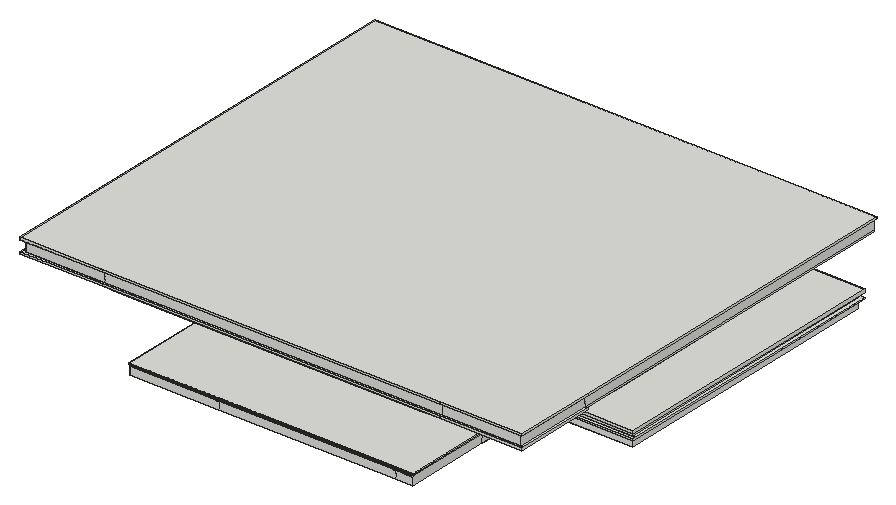
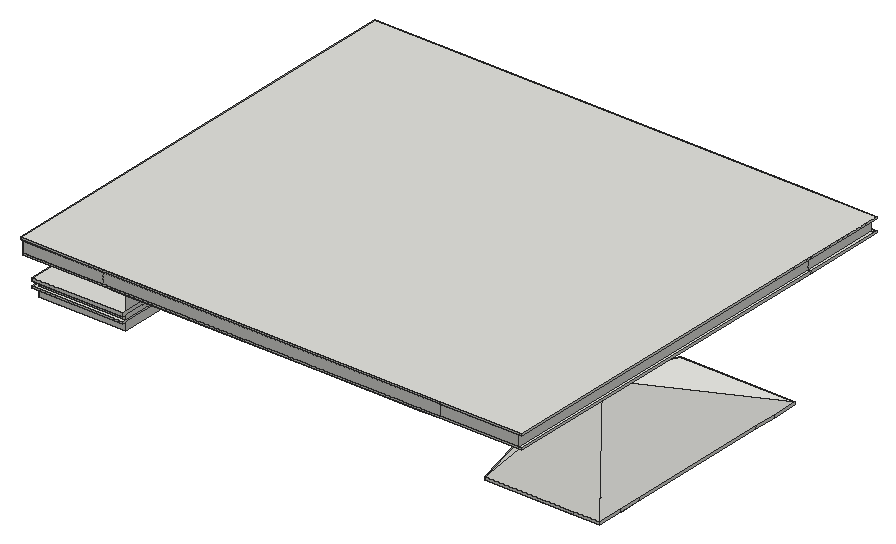
# SketchUp Ruby script. Lengths in inches.
U = 1.inch
M = Sketchup.active_model
def pt(a) = Geom::Point3d.new(a.map { |v| v * U })
def face(e, loops, mat)
  f = e.add_face(loops[0].map { |a| pt(a) })
  loops[1..].each { |l| e.add_face(l.map { |a| pt(a) }).erase! }
  f.material = f.back_material = mat if mat
  f
end
# faces: each face lists its corners as indices into pts; further lists are holes
def faces(e, pts, list, mat = nil) = list.each { |f| face(e, (f[0].is_a?(Array) ? f : [f]).map { |l| l.map { |i| pts[i] } }, mat) }
# xy, xz, yz: faces in a plane at the given z, y or x. An outline is a flat list of corners, or four numbers for a rectangle; further outlines are holes
def ring(l) = l.size == 4 ? [[l[0], l[1]], [l[2], l[1]], [l[2], l[3]], [l[0], l[3]]] : l.each_slice(2).to_a
def flat(e, list, mat, &to3) = list.each { |f| face(e, (f[0].is_a?(Array) ? f : [f]).map { |l| ring(l).map { |u, v| to3.(u, v) } }, mat) }
def xy(e, z, list, mat = nil) = flat(e, list, mat) { |x, y| [x, y, z] }
def xz(e, y, list, mat = nil) = flat(e, list, mat) { |x, z| [x, y, z] }
def yz(e, x, list, mat = nil) = flat(e, list, mat) { |y, z| [x, y, z] }
def lines(e, pts, list) = list.each { |a, b| e.add_line(pt(pts[a]), pt(pts[b])) }
# prism: a flat outline (further loops are holes) pulled along v
def prism(e, loops, v, mat = nil)
  f = face(e, loops, mat); d = Geom::Vector3d.new(v.map { |x| x * U })
  f.pushpull(f.normal.samedirection?(d) ? d.length : -d.length)
end
def box(e, o, s, mat = nil) = prism(e, [[o, [o[0] + s[0], o[1], o[2]], [o[0] + s[0], o[1] + s[1], o[2]], [o[0], o[1] + s[1], o[2]]]], [0, 0, s[2]], mat)
def at(x, y, z, deg = 0) = Geom::Transformation.translation(pt([x, y, z])) * Geom::Transformation.rotation(ORIGIN, Z_AXIS, deg.degrees)
def axes(o, x, y, z) = Geom::Transformation.new([*x, 0, *y, 0, *z, 0, *pt(o).to_a, 1])
def part(name) = M.definitions.add(name)
# library, detail: a bought-in or finely detailed component or shape, given as its bounding box
def library(name, o, s) = part(name).tap { |d| box(d.entities, o, s) }
def detail(e, o, s) = box(e.add_group.entities, o, s)
def put(e, d, t, mat = nil) = e.add_instance(d, t).tap { |i| i.material = mat if mat }
def group(e, t, mat = nil) = e.add_group.tap { |g| g.transformation = t; g.material = mat if mat }.entities
root = M.entities
M.materials.add("Glass Thin Clear 001").color = [255, 250, 250]
M.materials["Glass Thin Clear 001"].alpha = 0.1
M.materials.add("[Color M07]").color = [58, 58, 58]
xy(root,335.4,[[79.0625,304.1875,79.0625,318.3125,79.875,318.3125,79.875,305,93.1875,305,93.1875,304.1875],[93.1875,304.1875,94,305],[94,304.1875,142,305],[79.875,305,93.1875,318.3125],[93.1875,305,94,318.3125],
  [94,305,142,318.3125],[79.0625,318.3125,79.875,331.125],[79.875,318.3125,93.1875,319.125],[93.1875,318.3125,94,319.125],[94,318.3125,142,319.125],
  [79.875,319.125,93.1875,331.125],[93.1875,319.125,94,331.125],[94,319.125,142,423.25],[79.0625,331.125,79.875,411.25],[79.875,331.125,93.1875,411.25],
  [93.1875,331.125,94,411.25],[79.0625,411.25,79.875,423.25],[79.875,411.25,93.1875,423.25],[93.1875,411.25,94,423.25],[79.0625,423.25,79.875,424.0625],
  [79.875,423.25,93.1875,424.0625],[93.1875,423.25,94,424.0625],[94,423.25,142,424.0625],[79.0625,424.0625,79.0625,438.1875,93.1875,438.1875,93.1875,437.375,79.875,437.375,79.875,424.0625],[79.875,424.0625,93.1875,437.375],
  [93.1875,424.0625,94,437.375],[94,424.0625,142,437.375],[93.1875,437.375,142,438.1875]])
xy(root,350.5625,[[326.84,298.82,374.84,453.63]])
xy(root,351.07,[[169.81,269.93,207.43,270.37],[169.81,270.37,207.43,272.05]],"[Color M07]")
xy(root,351.46,[[241.62,260.1875,243.38,264.4375],[261.3,260.1875,263.07,264.4375],[283.05,260.1875,284.82,264.4375],[308.3125,260.1875,310.08,264.4375]])
xy(root,351.46,[[223.93,260.1875,241.62,261.1875],[243.38,260.1875,261.3,261.1875],[263.07,260.1875,283.05,261.1875],[284.82,260.1875,308.3125,261.1875],[310.08,260.1875,317.84,261.1875],
  [317.84,260.1875,323.73,261.1875],[223.93,261.1875,241.62,264.4375],[243.38,261.1875,261.3,264.4375],[263.07,261.1875,283.05,264.4375],[284.82,261.1875,308.3125,264.4375],
  [310.08,261.1875,317.84,264.4375],[317.84,261.1875,323.73,264.4375]],"[Color M07]")
xy(root,354.57,[[171.8125,207.6875,220.8125,255.6875],[220.8125,207.6875,317.84,255.6875],[317.84,207.6875,326.84,255.6875],[171.8125,255.6875,209.4375,264.6875],[220.8125,255.6875,317.84,260.1875],
  [317.84,255.6875,326.84,260.1875],[220.8125,264.4375,317.84,264.6875],[317.84,264.4375,326.84,264.6875],[171.8125,264.6875,171.8125,271.43,173.3125,271.43,173.3125,269.93,209.4375,269.93,209.4375,264.6875],[171.8125,271.43,171.8125,280.43,209.4375,280.43,209.4375,272.05,173.3125,272.05,173.3125,271.43]])
xy(root,354.57,[[220.8125,260.1875,317.84,262.625],[317.84,260.1875,326.84,262.625],[220.8125,262.625,317.84,264.4375],[317.84,262.625,326.84,264.4375],[173.3125,269.93,209.4375,271.43],
  [209.4375,269.93,210.9375,271.43],[173.3125,271.43,209.4375,272.05],[209.4375,271.43,210.9375,272.05]],"[Color M07]")
xy(root,354.9375,[[326.84,296.95,376.71,298.82],[326.84,298.82,374.84,453.63],[374.84,298.82,376.71,455.51],[326.84,453.63,374.84,455.51]])
xy(root,355.8125,[[326.84,296.95,376.71,298.82],[326.84,298.82,374.84,453.63],[374.84,298.82,376.71,455.51],[326.84,453.63,374.84,455.51]])
xy(root,356.5,[[169.62,269.93,169.81,270.37],[169.62,270.37,169.81,272.05]],"[Color M07]")
xy(root,356.87,[[166.4375,269.93,168.4375,272.05]])
xy(root,356.87,[[145.94,269.93,166.4375,270.37],[168.4375,269.93,169.62,270.37],[145.94,270.37,166.4375,272.05],[168.4375,270.37,169.62,272.05]],"[Color M07]")
xy(root,357.54,[[142,273.2,142.4375,280.43],[142.4375,273.2,144.125,280.43],[142,280.43,142.4375,289.29],[142.4375,280.43,144.125,289.29]],"[Color M07]")
xy(root,358.3125,[[326.84,296.95,376.71,298.82],[326.84,298.82,374.84,453.63],[374.84,298.82,376.71,455.51],[326.84,453.63,374.84,455.51]])
xy(root,359,[[171.625,207.5625,171.8125,280.43],[171.8125,207.5625,220.8125,207.6875],[220.8125,207.5625,317.84,207.6875],[317.84,207.5625,326.84,207.6875]])
xy(root,359.1875,[[171.8125,207.6875,326.84,255.6875]])
xy(root,359.4375,[[171.625,207.5625,209.5625,207.5625,209.5625,207.8125,171.9375,207.8125,171.9375,255.6875,171.8125,255.6875,171.8125,280.43,171.625,280.43],[209.5625,207.5625,220.8125,207.8125],[220.8125,207.5625,317.84,207.8125],[317.84,207.5625,326.84,207.8125],[171.9375,207.8125,326.71,255.6875],
  [326.71,207.8125,326.84,255.6875]])
xy(root,360,[[171.625,207.5,171.625,271.43,171.8125,271.43,171.8125,255.6875,171.9375,255.6875,171.9375,207.8125,209.5625,207.8125,209.5625,207.5],[209.5625,207.5,220.8125,207.8125],[220.8125,207.5,317.84,207.8125],[317.84,207.5,327.03,207.8125],[171.9375,207.8125,326.71,255.6875],
  [326.71,207.8125,327.03,255.6875],[171.8125,255.6875,171.9375,264.6875],[171.9375,255.6875,326.84,264.6875],[171.8125,264.6875,171.9375,271.43],[171.9375,264.6875,171.9375,271.43,173.125,271.43,173.125,269.93,173.3125,269.93,173.3125,271.43,220.8125,271.43,220.8125,264.6875],
  [220.8125,264.6875,317.84,271.43],[317.84,264.6875,326.84,271.43],[171.625,271.43,171.8125,280.43],[326.84,296.95,376.71,455.51]])
xy(root,360,[[173.125,269.93,173.3125,271.43],[173.125,271.43,173.3125,272.05]],"[Color M07]")
xy(root,360.375,[[171.625,271.43,173.125,272.05],[173.25,271.43,209.4375,272.18],[209.4375,271.43,211.0625,272.18],[211.0625,271.43,211.0625,272.18,209.4375,272.18,209.4375,280.43,220.8125,280.43,220.8125,271.43],[220.8125,271.43,326.84,280.43],
  [171.625,272.18,209.4375,280.43]])
xy(root,360.375,[[142,269.8,143.625,269.93],[143.625,269.8,144.375,269.93],[144.375,269.8,144.375,269.93,173.125,269.93,173.125,271.43,173.25,271.43,173.25,269.8],[173.25,269.8,211.0625,271.43],[142,269.93,143.5,271.43],
  [143.5,269.93,143.625,271.43],[143.625,269.93,144.125,271.43],[144.125,269.93,144.375,271.43],[144.375,269.93,173.125,271.43],[142,271.43,143.5,280.43],
  [143.5,271.43,143.625,280.43],[143.625,271.43,144.125,280.43],[144.125,271.43,144.375,272.05],[144.375,271.43,144.375,272.05,171.625,272.05,171.625,272.18,173.25,272.18,173.25,271.43,173.125,271.43,173.125,272.05,171.625,272.05,171.625,271.43],[144.125,272.05,144.375,280.43],
  [144.375,272.05,171.625,272.18],[142,280.43,143.5,292.12],[143.5,280.43,143.625,292.12],[143.625,280.43,144.125,292.12],[144.125,280.43,144.375,292.12]],"[Color M07]")
xy(root,360.6875,[[171.625,207.5,327.03,207.5,327.03,255.6875,326.84,255.6875,326.84,271.43,171.625,271.43]])
xy(root,361.53,[[142,271.52,142.5625,280.43],[142.5625,271.52,144.375,280.43],[142,280.43,142.5625,290.97],[142.5625,280.43,144.375,290.97]],"[Color M07]")
xy(root,361.68,[[143.86,269.8,144.375,270.37],[166.5625,269.8,168.5625,272.18]])
xy(root,361.68,[[144.375,269.8,166.5625,270.37],[168.5625,269.8,173.25,270.37],[173.25,269.8,209.76,270.37],[144.375,270.37,166.5625,272.18],[168.5625,270.37,173.25,272.18],
  [173.25,270.37,209.76,272.18]],"[Color M07]")
xy(root,366.64,[[143.86,269.8,144.375,270.37],[166.5625,269.8,168.5625,272.18]])
xy(root,366.64,[[144.375,269.8,166.5625,270.37],[168.5625,269.8,209.76,270.37],[144.375,270.37,166.5625,272.18],[168.5625,270.37,209.76,272.18]],"[Color M07]")
xy(root,366.79,[[142,271.52,142.5625,280.43],[142.5625,271.52,144.375,280.43],[142,280.43,142.5625,290.97],[142.5625,280.43,144.375,290.97]],"[Color M07]")
xy(root,367.9375,[[144.375,272.18,144.375,292.12,151,292.12,151,280.43,209.4375,280.43,209.4375,272.18]])
xy(root,367.9375,[[142,269.8,143.625,271.43],[143.625,269.8,144.375,271.43],[144.375,269.8,211.0625,271.43],[142,271.43,143.625,280.43],[143.625,271.43,144.375,280.43],
  [209.4375,271.43,211.0625,272.18],[142,280.43,143.625,292.12],[143.625,280.43,144.375,292.12]],"[Color M07]")
xy(root,379.5625,[[96.8125,226.24,142,271.43],[142,226.24,151,271.43],[151,226.24,209.4375,271.43],[209.4375,226.24,317.84,271.43],[317.84,226.24,326.84,271.43],
  [326.84,226.24,372.03,271.43],[96.8125,271.43,142,280.43],[142,271.43,151,280.43],[151,271.43,209.4375,280.43],[209.4375,271.43,317.84,280.43],
  [317.84,271.43,326.84,280.43],[326.84,271.43,370.4,280.43],[96.8125,280.43,142,292.12],[142,280.43,151,292.12],[151,280.43,209.4375,460.5625],
  [209.4375,280.43,209.4375,469.5625,317.84,469.5625,317.84,460.5625,220.8125,460.5625,220.8125,280.43],[220.8125,280.43,317.84,460.5625],[317.84,280.43,326.84,469.5625],[326.84,280.43,370.4,298.82],[96.8125,292.12,142,460.5625],
  [142,292.12,151,469.5625],[326.84,298.82,370.4,453.63],[326.84,453.63,370.4,469.5625],[96.8125,460.5625,142,469.5625],[151,460.5625,209.4375,469.5625]])
xy(root,380.6875,[[96.8125,226.24,142,227.87],[142,226.24,326.84,227.87],[326.84,226.24,372.03,227.87],[96.8125,227.87,98.4375,271.43],[98.4375,227.87,370.4,469.5625],
  [370.4,227.87,372.03,271.43],[96.8125,271.43,98.4375,469.5625]])
xy(root,386.6875,[[96.8125,226.24,98.4375,271.43],[98.4375,226.24,142,227.87],[142,226.24,326.84,227.87],[326.84,226.24,372.03,227.87],[98.4375,227.87,370.4,469.5625],
  [370.4,227.87,372.03,271.43],[96.8125,271.43,98.4375,469.5625],[370.4,271.43,372.03,469.5625]])
xy(root,387.75,[[96.8125,226.24,372.03,469.5625]])
xz(root,207.5,[[171.625,360,220.8125,360.6875],[220.8125,360,317.84,360.6875],[317.84,360,327.03,360.6875]])
xz(root,207.5625,[[171.625,359,220.8125,359.4375],[220.8125,359,317.84,359.4375],[317.84,359,326.84,359.4375]])
xz(root,207.6875,[[171.8125,354.57,220.8125,359],[220.8125,354.57,317.84,359],[317.84,354.57,326.84,359],[171.8125,359,220.8125,359.1875],[220.8125,359,317.84,359.1875],
  [317.84,359,326.84,359.1875]])
xz(root,207.8125,[[171.9375,359.4375,220.8125,360],[220.8125,359.4375,317.84,360],[317.84,359.4375,326.71,360]])
xz(root,226.24,[[96.8125,379.5625,142,380.6875],[142,379.5625,326.84,380.6875],[326.84,379.5625,372.03,380.6875],[96.8125,386.6875,142,387.75],[142,386.6875,326.84,387.75],
  [326.84,386.6875,372.03,387.75]])
xz(root,227.87,[[98.4375,380.6875,142,386.6875],[142,380.6875,326.84,386.6875],[326.84,380.6875,370.4,386.6875]])
xz(root,255.6875,[[171.8125,354.57,220.8125,359.1875],[220.8125,354.57,317.84,359.1875],[317.84,354.57,326.84,359.1875],[171.8125,359.1875,220.8125,359.4375],[220.8125,359.1875,317.84,359.4375],
  [317.84,359.1875,326.84,359.4375],[171.8125,359.4375,171.9375,360],[171.9375,359.4375,220.8125,360],[220.8125,359.4375,317.84,360],[317.84,359.4375,326.71,360],
  [326.71,359.4375,326.84,360],[326.84,360,327.03,360.6875]])
xz(root,264.6875,[[220.8125,354.57,317.84,360],[317.84,354.57,326.84,360]])
xz(root,269.8,[[142,360.375,144.375,360.375,144.375,361.68,143.86,361.68,143.86,366.64,144.375,366.64,144.375,367.9375,142,367.9375],[144.375,360.375,211.0625,360.375,211.0625,367.9375,144.375,367.9375,144.375,366.64,209.76,366.64,209.76,361.68,144.375,361.68],[143.86,361.68,144.375,366.64],[166.5625,361.68,168.5625,366.64]],"[Color M07]")
xz(root,270.37,[[143.86,361.68,166.5625,366.64],[168.5625,361.68,209.76,366.64]],"Glass Thin Clear 001")
xz(root,271.43,[[171.8125,354.57,173.3125,360],[173.3125,354.57,209.4375,360],[171.625,360,173.125,360.375],[173.125,360,209.4375,360.375],[209.4375,360,220.8125,360.375],
  [220.8125,360,317.84,360.375],[317.84,360,326.84,360.375],[142.5625,360.375,143.625,367.9375],[171.625,360.375,209.4375,360.6875],[209.4375,360.375,211.0625,360.6875],
  [211.0625,360.375,220.8125,360.6875],[220.8125,360.375,317.84,360.6875],[317.84,360.375,326.84,360.6875],[211.0625,360.6875,317.84,360.6875,317.84,379.5625,202,379.5625,202,367.9375,211.0625,367.9375],[317.84,360.6875,326.84,379.5625],
  [142,367.9375,202,379.5625],[370.4,379.5625,372.03,380.6875]])
xz(root,271.43,[[143.625,360.375,143.625,367.9375,209.4375,367.9375,209.4375,360.6875,171.625,360.6875,171.625,360.375],[209.4375,360.6875,211.0625,367.9375]],"Glass Thin Clear 001")
xz(root,271.52,[[142,361.53,142.5625,366.79],[142.5625,361.53,144.375,366.79]],"[Color M07]")
xz(root,272.18,[[144.375,360.375,144.375,361.68,209.76,361.68,209.76,366.64,144.375,366.64,144.375,367.9375,211.0625,367.9375,211.0625,360.375],[166.5625,361.68,168.5625,366.64]],"[Color M07]")
xz(root,280.43,[[171.8125,354.57,171.8125,359,171.625,359,171.625,359.4375,171.8125,359.4375,171.8125,360,171.625,360,171.625,360.375,209.4375,360.375,209.4375,354.57],[209.4375,360.375,220.8125,379.5625],[220.8125,360.375,326.84,379.5625],[151,367.9375,209.4375,379.5625]])
xz(root,290.97,[[142,361.53,142.5625,366.79],[142.5625,361.53,144.375,366.79]],"[Color M07]")
xz(root,292.12,[[144.375,360.375,151,367.9375],[142,367.9375,151,379.5625]])
xz(root,292.12,[[142,360.375,143.625,367.9375],[143.625,360.375,144.375,367.9375]],"[Color M07]")
xz(root,296.95,[[326.84,354.9375,376.71,355.8125],[326.84,358.3125,376.71,360]])
xz(root,298.82,[[326.84,350.5625,374.84,354.9375],[326.84,355.8125,374.84,358.3125]])
xz(root,304.1875,[[79.0625,335.4,93.1875,336.97],[93.1875,335.4,142,336.97]])
xz(root,438.1875,[[79.0625,335.4,93.1875,336.97],[93.1875,335.4,142,336.97]])
xz(root,453.63,[[326.84,350.5625,374.84,354.9375],[326.84,355.8125,374.84,358.3125]])
xz(root,455.51,[[326.84,354.9375,376.71,355.8125],[326.84,358.3125,376.71,360]])
xz(root,469.5625,[[96.8125,379.5625,142,380.6875],[142,379.5625,326.84,380.6875],[326.84,379.5625,370.4,380.6875],[98.4375,380.6875,142,386.6875],[142,380.6875,326.84,386.6875],
  [326.84,380.6875,370.4,386.6875],[96.8125,386.6875,142,387.75],[142,386.6875,326.84,387.75],[326.84,386.6875,372.03,387.75]])
yz(root,79.0625,[[304.1875,335.4,318.3125,336.97],[318.3125,335.4,331.125,336.97],[331.125,335.4,411.25,336.97],[411.25,335.4,424.0625,336.97],[424.0625,335.4,438.1875,336.97]])
yz(root,96.8125,[[226.24,379.5625,271.43,380.6875],[271.43,379.5625,469.5625,380.6875],[226.24,386.6875,271.43,387.75],[271.43,386.6875,469.5625,387.75]])
yz(root,98.4375,[[227.87,380.6875,271.43,386.6875],[271.43,380.6875,469.5625,386.6875]])
yz(root,142,[[304.1875,335.4,318.3125,336.97],[318.3125,335.4,331.125,336.97],[331.125,335.4,411.25,335.4,411.25,336.97,371.1875,359.28,331.125,336.97],[411.25,335.4,424.0625,336.97],[424.0625,335.4,438.1875,336.97],
  [304.1875,336.97,371.1875,359.28,331.125,336.97],[411.25,336.97,371.1875,359.28,438.1875,336.97],[271.43,367.9375,292.12,379.5625]])
yz(root,142,[[[269.8,360.375,292.12,367.9375],[271.52,361.53,290.97,366.79]]],"[Color M07]")
yz(root,142.5625,[[271.52,361.53,290.97,366.79]],"Glass Thin Clear 001")
yz(root,143.625,[[271.43,360.375,292.12,367.9375]],"Glass Thin Clear 001")
yz(root,143.86,[[269.8,361.68,270.37,366.64]])
yz(root,144.375,[[269.8,360.375,272.18,360.375,272.18,361.53,271.52,361.53,271.52,361.68,269.8,361.68],[269.8,366.64,271.52,366.64,271.52,366.79,272.18,366.79,272.18,367.9375,269.8,367.9375]])
yz(root,144.375,[[272.18,360.375,292.12,360.375,292.12,367.9375,272.18,367.9375,272.18,366.79,290.97,366.79,290.97,361.53,272.18,361.53],[271.52,361.53,272.18,361.68],[269.8,361.68,271.52,366.64],[271.52,366.64,272.18,366.79]],"[Color M07]")
yz(root,151,[[280.43,367.9375,292.12,379.5625]])
yz(root,166.5625,[[269.8,361.68,270.37,366.64],[270.37,361.68,272.18,366.64]],"[Color M07]")
yz(root,168.5625,[[269.8,361.68,270.37,366.64],[270.37,361.68,272.18,366.64]],"[Color M07]")
yz(root,169.62,[[269.93,356.5,270.37,356.87],[270.37,356.5,272.05,356.87]],"[Color M07]")
yz(root,169.81,[[269.93,351.07,270.37,356.5],[270.37,351.07,272.05,356.5]],"[Color M07]")
yz(root,171.625,[[207.5625,359,280.43,359.4375],[207.5,360,271.43,360.6875],[271.43,360,280.43,360.375]])
yz(root,171.8125,[[207.6875,354.57,255.6875,359],[255.6875,354.57,264.6875,359],[264.6875,354.57,271.43,359],[271.43,354.57,280.43,359],[207.6875,359,255.6875,359.1875],
  [255.6875,359,264.6875,359.1875],[264.6875,359,271.43,359.1875],[255.6875,359.1875,264.6875,359.4375],[264.6875,359.1875,271.43,359.4375],[255.6875,359.4375,264.6875,360],
  [264.6875,359.4375,271.43,360],[271.43,359.4375,280.43,360]])
yz(root,171.9375,[[207.8125,359.4375,255.6875,360]])
yz(root,173.125,[[269.93,360,271.43,360.375],[271.43,360,272.05,360.375]],"[Color M07]")
yz(root,173.3125,[[269.93,354.57,271.43,360],[271.43,354.57,272.05,360]],"[Color M07]")
yz(root,209.4375,[[271.43,354.57,280.43,360.375],[271.43,360.375,280.43,367.9375]])
yz(root,209.76,[[269.8,361.68,270.37,366.64],[270.37,361.68,272.18,366.64]],"[Color M07]")
yz(root,211.0625,[[269.8,360.375,271.43,367.9375],[271.43,360.375,272.18,367.9375]],"[Color M07]")
yz(root,326.71,[[207.8125,359.4375,255.6875,360]])
yz(root,326.84,[[298.82,350.5625,453.63,354.9375],[207.6875,354.57,255.6875,359.1875],[255.6875,354.57,264.6875,360],[296.95,354.9375,455.51,355.8125],[298.82,355.8125,453.63,358.3125],
  [296.95,358.3125,455.51,360],[207.5625,359,207.6875,359,207.6875,359.1875,255.6875,359.1875,255.6875,359.4375,207.5625,359.4375],[255.6875,360,271.43,360.6875],[298.82,360,453.63,379.5625],[271.43,360.375,280.43,379.5625]])
yz(root,327.03,[[207.5,360,255.6875,360.6875]])
yz(root,370.4,[[271.43,379.5625,469.5625,380.6875],[227.87,380.6875,271.43,386.6875],[271.43,380.6875,469.5625,386.6875]])
yz(root,372.03,[[226.24,379.5625,271.43,380.6875],[226.24,386.6875,271.43,387.75],[271.43,386.6875,469.5625,387.75]])
yz(root,374.84,[[298.82,350.5625,453.63,354.9375],[298.82,355.8125,453.63,358.3125]])
yz(root,376.71,[[296.95,354.9375,455.51,355.8125],[296.95,358.3125,455.51,360]])
p = [[79.0625,304.1875,336.97],[93.1875,304.1875,336.97],[142,304.1875,336.97],[130.9375,371.1875,359.28],[79.0625,438.1875,336.97],[79.0625,424.0625,336.97],
  [79.0625,411.25,336.97],[79.0625,331.125,336.97],[79.0625,318.3125,336.97],[142,371.1875,359.28],[142,438.1875,336.97],[93.1875,438.1875,336.97],
  [317.84,280.43,360.375],[317.84,280.43,360],[317.84,271.43,360],[326.84,271.43,379.5625],[326.84,271.43,385.5625],[93.1875,424.0625,336.97],
  [93.1875,424.0625,335.4],[93.1875,411.25,336.97],[93.1875,411.25,335.4],[93.1875,331.125,335.4],[93.1875,331.125,336.97]]
faces(root,p,[[0,1,2,3],[0,3,4,5,6,7,8],[3,2,9],[4,3,10,11],[3,9,10]])
lines(root,p,[[12,13],[13,14],[15,16],[17,18],[19,20],[21,22]])
